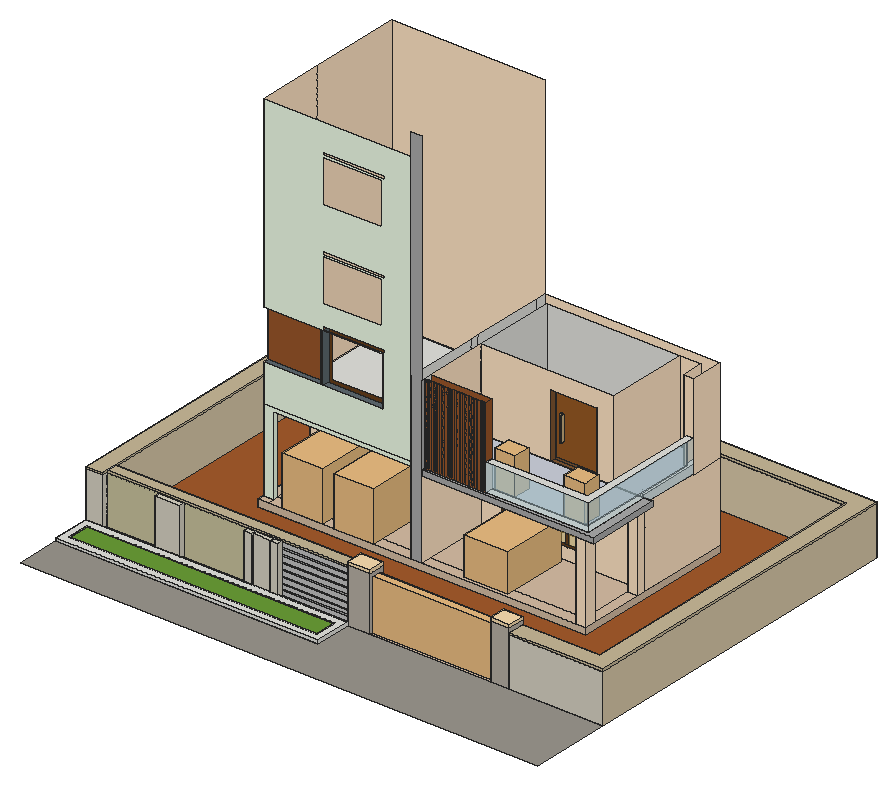
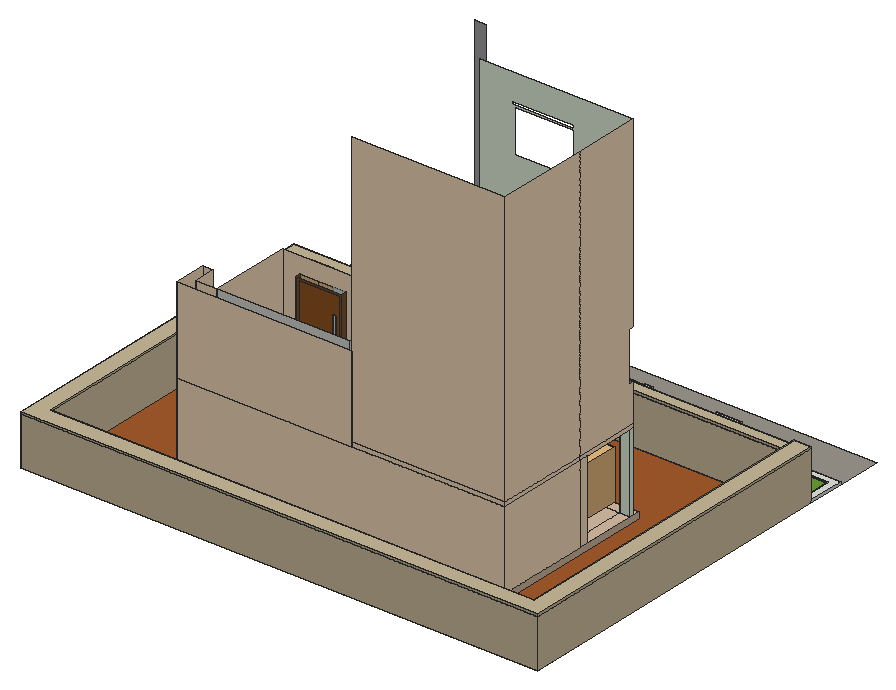
# SketchUp Ruby script. Lengths in inches.
U = 1.inch
M = Sketchup.active_model
def pt(a) = Geom::Point3d.new(a.map { |v| v * U })
def face(e, loops, mat)
  f = e.add_face(loops[0].map { |a| pt(a) })
  loops[1..].each { |l| e.add_face(l.map { |a| pt(a) }).erase! }
  f.material = f.back_material = mat if mat
  f
end
# faces: each face lists its corners as indices into pts; further lists are holes
def faces(e, pts, list, mat = nil) = list.each { |f| face(e, (f[0].is_a?(Array) ? f : [f]).map { |l| l.map { |i| pts[i] } }, mat) }
# xy, xz, yz: faces in a plane at the given z, y or x. An outline is a flat list of corners, or four numbers for a rectangle; further outlines are holes
def ring(l) = l.size == 4 ? [[l[0], l[1]], [l[2], l[1]], [l[2], l[3]], [l[0], l[3]]] : l.each_slice(2).to_a
def flat(e, list, mat, &to3) = list.each { |f| face(e, (f[0].is_a?(Array) ? f : [f]).map { |l| ring(l).map { |u, v| to3.(u, v) } }, mat) }
def xy(e, z, list, mat = nil) = flat(e, list, mat) { |x, y| [x, y, z] }
def xz(e, y, list, mat = nil) = flat(e, list, mat) { |x, z| [x, y, z] }
def yz(e, x, list, mat = nil) = flat(e, list, mat) { |y, z| [x, y, z] }
def lines(e, pts, list) = list.each { |a, b| e.add_line(pt(pts[a]), pt(pts[b])) }
# prism: a flat outline (further loops are holes) pulled along v
def prism(e, loops, v, mat = nil)
  f = face(e, loops, mat); d = Geom::Vector3d.new(v.map { |x| x * U })
  f.pushpull(f.normal.samedirection?(d) ? d.length : -d.length)
end
def box(e, o, s, mat = nil) = prism(e, [[o, [o[0] + s[0], o[1], o[2]], [o[0] + s[0], o[1] + s[1], o[2]], [o[0], o[1] + s[1], o[2]]]], [0, 0, s[2]], mat)
def at(x, y, z, deg = 0) = Geom::Transformation.translation(pt([x, y, z])) * Geom::Transformation.rotation(ORIGIN, Z_AXIS, deg.degrees)
def axes(o, x, y, z) = Geom::Transformation.new([*x, 0, *y, 0, *z, 0, *pt(o).to_a, 1])
def part(name) = M.definitions.add(name)
# library, detail: a bought-in or finely detailed component or shape, given as its bounding box
def library(name, o, s) = part(name).tap { |d| box(d.entities, o, s) }
def detail(e, o, s) = box(e.add_group.entities, o, s)
def put(e, d, t, mat = nil) = e.add_instance(d, t).tap { |i| i.material = mat if mat }
def group(e, t, mat = nil) = e.add_group.tap { |g| g.transformation = t; g.material = mat if mat }.entities
root = M.entities
M.materials.add("[0012_Bisque]").color = [255, 228, 196]
M.materials.add("[Carrera Marble]").color = [193, 193, 193]
M.materials.add("[Color M03]").color = [170, 170, 170]
M.materials.add("[Field Square Tile]").color = [217, 201, 169]
M.materials.add("[Formica Beige]").color = [249, 221, 176]
M.materials.add("[Formica Graystone]").color = [214, 209, 194]
M.materials.add("[Formica Laminate Light]").color = [213, 189, 164]
M.materials.add("[Formica Speckled Grey]1").color = [94, 105, 111]
M.materials.add("[Grass Dark Green]").color = [106, 157, 55]
M.materials.add("[Marble Carrara Floor Tile]").color = [204, 208, 219]
M.materials.add("[Quartz Light Brown]").color = [199, 184, 152]
M.materials.add("[Quartz Light Grey]").color = [251, 251, 252]
M.materials.add("[Rough Square Concrete Block]").color = [155, 151, 142]
M.materials.add("[Stone Coursed Rough]").color = [201, 195, 158]
M.materials.add("[Stone Masonry Multi]").color = [182, 175, 164]
M.materials.add("[Tile Limestone Large]1").color = [238, 251, 230]
M.materials.add("[Translucent Glass Gray]").color = [221, 178, 79]
M.materials["[Translucent Glass Gray]"].alpha = 0.5
M.materials.add("[Translucent Glass Safety]").color = [204, 235, 244]
M.materials["[Translucent Glass Safety]"].alpha = 0.42
M.materials.add("[Wood Bamboo]").color = [150, 89, 36]
M.materials.add("[Wood Cherry Original]").color = [152, 86, 42]
M.materials.add("[Wood Floor Light]").color = [204, 176, 127]
M.materials.add("[Wood Floor Parquet]").color = [102, 62, 27]
M.materials.add("[Wood Floor]").color = [127, 86, 50]
M.materials.add("[Wood Square Tile 01]").color = [164, 91, 44]
M.materials.add("[Wood Veneer 01]").color = [89, 52, 27]
M.materials.add("[Wood Veneer 02]").color = [119, 80, 57]
M.materials.add("[Wood Veneer 02]1").color = [190, 128, 91]
c1 = library("Gate_Lasercut_10ftx6ft_Kalil",[-0.15,-3.25,-0.15],[120,5.625,60.3])
c2 = library("skpE847",[-111.76,-15.01,0.76],[2.12,4.6,1.82])
c3 = part("car+1")
p = [[0,0,0],[1,0,0],[1,1,0]]
lines(c3.entities,p,[[0,1],[1,2],[2,0]])
put(c3.entities,c2,axes([-477.97,5140.8,-31.25],[0,46,0],[-46,0,0],[0,0,40.94]))
c4 = library("2015 Porsche Macan",[0.14,0.6,0.32],[90.05,184.43,65.58])
c5 = library("chau cay",[-24.34,-109.24,0],[56.46,62.58,79.69])
xy(root,0,[[[0,283.68,1655,516.81],[43.91,327.6,1611.08,472.9]],[0,516.81,0,2678.22,3268.59,2678.22,3268.59,516.81,2676.2,516.81,2676.2,622.2,3163.2,622.2,3163.2,2572.82,105.39,2572.82,105.39,516.81],[437.72,516.81,594.8,552.32],[997.32,516.81,1049.71,552.32],[1165.48,516.81,1213.51,552.32],
  [1655,516.81,1796.11,622.2],[2557.88,516.81,2676.2,622.2],[1049.71,525.25,1165.48,552.32],[105.39,552.32,1655,622.2],[560.3125,1175.74,2634.5,2234.7]])
xy(root,0,[[1796.11,516.81,2557.88,622.2]],"[Formica Laminate Light]")
xy(root,0,[[105.39,516.81,437.72,552.32],[594.8,516.81,997.32,552.32],[1049.71,516.81,1165.48,525.25],[1213.51,516.81,1655,552.32]],"[Quartz Light Grey]")
xy(root,0,[[0,0,0,283.68,1655,283.68,1655,516.81,3268.59,516.81,3268.59,0]],"[Rough Square Concrete Block]")
xy(root,0,[[[105.39,622.2,3163.2,2572.82],[560.3125,1175.74,2634.5,2234.7]]],"[Wood Square Tile 01]")
xy(root,12.4375,[[43.91,327.6,1611.08,472.9]],"[Grass Dark Green]")
xy(root,19,[[[0,283.68,1655,516.81],[43.91,327.6,1611.08,472.9]]])
xy(root,42.38,[[1529,1175.74,1597.41,1644.77],[2570.48,1175.74,2634.5,1247.68],[560.3125,1221.52,624.34,1247.68],[1504.0625,1221.52,1529,1247.68],[1504.0625,1247.68,1529,1644.77],
  [560.3125,1583.4,624.34,1644.77],[2570.48,1583.4,2634.5,1644.77],[560.3125,1644.77,560.3125,2234.7,2634.5,2234.7,2634.5,1644.77,2570.48,1644.77,2570.48,2162.77,624.34,2162.77,624.34,1644.77],[624.34,1644.77,624.34,1705.22,2570.48,1705.22,2570.48,1644.77,1498.82,1644.77,1498.82,1683.34,1254.8,1683.34,1254.8,1644.77],[624.34,1705.22,2570.48,2162.77]])
xy(root,42.38,[[560.3125,1175.74,624.34,1221.52],[624.34,1175.74,1529,1175.74,1529,1221.52,1504.0625,1221.52,1504.0625,1247.68,624.34,1247.68],[1597.41,1175.74,2570.48,1247.68],[560.3125,1247.68,624.34,1583.4],[624.34,1247.68,1504.0625,1247.68,1504.0625,1644.77,1498.82,1644.77,1498.82,1683.34,1254.8,1683.34,1254.8,1644.77,624.34,1644.77],
  [1597.41,1247.68,2570.48,1644.77],[2570.48,1247.68,2634.5,1583.4]],"[Formica Laminate Light]")
xy(root,305.6875,[[0,516.81,0,2678.22,3268.59,2678.22,3268.59,516.81,2676.2,516.81,2676.2,622.2,3163.2,622.2,3163.2,2572.82,105.39,2572.82,105.39,516.81],[105.39,552.32,1655,622.2]])
xy(root,305.6875,[[437.72,516.81,594.8,552.32],[997.32,516.81,1049.71,552.32],[1165.48,516.81,1213.51,552.32],[1049.71,525.25,1165.48,552.32]],"[Formica Graystone]")
xy(root,318.25,[[0,516.81,105.39,516.81,105.39,2572.82,3163.2,2572.82,3163.2,622.2,2676.2,622.2,2676.2,516.81,3268.59,516.81,3268.59,2678.22,0,2678.22],[105.39,552.32,1655,622.2]],"[Quartz Light Brown]")
xy(root,342.3125,[[1655,516.81,1796.11,622.2],[2557.88,516.81,2676.2,622.2]])
xy(root,362.6875,[[1655,516.81,1796.11,622.2],[2557.88,516.81,2676.2,622.2]],"[Formica Beige]")
xy(root,463.2,[[1254.8,1644.77,1498.82,1683.34]],"[0012_Bisque]")
xy(root,535.87,[[2570.48,1175.74,2634.5,1247.68],[2634.5,1175.74,2683.95,1247.68],[560.3125,1583.4,560.3125,2234.7,1529,2234.7,1529,1644.77,624.34,1644.77,624.34,1583.4],[2570.48,1583.4,2634.5,1644.77],[2634.5,1583.4,2683.95,1644.77],
  [1597.41,1644.77,2570.48,2162.77]])
xy(root,535.87,[[1597.41,1175.74,1597.41,1644.77,2570.48,1644.77,2570.48,1583.4,2683.95,1583.4,2683.95,1247.68,2570.48,1247.68,2570.48,1175.74],[624.34,1221.52,1504.0625,1644.77]],"[0012_Bisque]")
xy(root,535.87,[[560.3125,1247.68,624.34,1583.4]],"[Tile Limestone Large]1")
xy(root,561.43,[[560.3125,1221.52,1529,2234.7]])
xy(root,569.39,[[1597.41,1197.49,1985.07,1247.68],[1985.07,1197.49,1985.07,1247.68,2590.83,1247.68,2590.83,1644.77,2634.5,1644.77,2634.5,1197.49],[1597.41,1644.77,1597.41,2162.77,2438.87,2162.77,2438.87,1644.77,2328.14,1644.77,2328.14,1674.71,2038.61,1674.71,2038.61,1644.77]])
xy(root,569.39,[[1597.41,1175.74,2683.95,1175.74,2683.95,1644.77,2634.5,1644.77,2634.5,1197.49,1597.41,1197.49]],"[Color M03]")
xy(root,569.39,[[1597.41,1247.68,2590.83,1644.77],[2438.87,1644.77,2590.83,1644.77,2590.83,2027.6,2570.48,2027.6,2570.48,2162.77,2438.87,2162.77]],"[Marble Carrara Floor Tile]")
xy(root,569.39,[[2038.61,1644.77,2328.14,1674.71]],"[Wood Floor]")
xy(root,740.5625,[[1985.07,1197.49,2634.5,1197.49,2634.5,2027.6,2590.83,2027.6,2590.83,1247.68,1985.07,1247.68]])
xy(root,798.61,[[560.3125,1221.52,922.73,1257.65],[937.5625,1221.52,1314.8125,1263.33]],"[Formica Speckled Grey]1")
xz(root,283.68,[[0,0,1655,19]])
xz(root,327.6,[[43.91,12.4375,1611.08,19]])
xz(root,327.6,[[43.91,0,1611.08,12.4375]],"[Grass Dark Green]")
xz(root,472.9,[[43.91,12.4375,1611.08,19]])
xz(root,472.9,[[43.91,0,1611.08,12.4375]],"[Grass Dark Green]")
xz(root,516.81,[[0,0,105.39,19],[105.39,0,437.72,19],[437.72,0,594.8,19],[594.8,0,997.32,19],[997.32,0,1049.71,19],
  [1049.71,0,1165.48,19],[1165.48,0,1213.51,19],[1213.51,0,1655,19]])
xz(root,516.81,[[1655,342.3125,1796.11,362.6875],[2557.88,342.3125,2676.2,362.6875]],"[Formica Beige]")
xz(root,516.81,[[2676.2,0,3268.59,305.6875],[0,19,105.39,305.6875],[437.72,19,594.8,305.6875],[997.32,19,1049.71,305.6875],[1165.48,19,1213.51,305.6875]],"[Formica Graystone]")
xz(root,516.81,[[0,305.6875,105.39,318.25],[2676.2,305.6875,3268.59,318.25]],"[Quartz Light Brown]")
xz(root,516.81,[[1655,0,1796.11,342.3125],[2557.88,0,2676.2,342.3125]],"[Stone Masonry Multi]")
xz(root,525.25,[[1049.71,0,1165.48,305.6875]],"[Formica Graystone]")
xz(root,552.32,[[437.72,0,594.8,305.6875],[997.32,0,1049.71,305.6875],[1049.71,0,1165.48,305.6875],[1165.48,0,1213.51,305.6875]])
xz(root,552.32,[[1213.51,0,1655,29.67],[1213.51,36.26,1655,62.625],[1213.51,69.17,1655,102.125],[1213.51,108.61,1655,141.5625],[1213.51,151.05,1655,184],
  [1213.51,191.55,1655,224.5],[1213.51,232.55,1655,265.5],[1213.51,272.74,1655,305.6875]],"[Carrera Marble]")
xz(root,552.32,[[1213.51,29.67,1655,36.26],[1213.51,62.625,1655,69.17],[1213.51,102.125,1655,108.61],[1213.51,141.5625,1655,151.05],[1213.51,184,1655,191.55],
  [1213.51,224.5,1655,232.55],[1213.51,265.5,1655,272.74]],"[Color M03]")
xz(root,552.32,[[105.39,305.6875,1655,318.25]],"[Quartz Light Brown]")
xz(root,552.32,[[105.39,0,437.72,305.6875],[594.8,0,997.32,305.6875]],"[Stone Coursed Rough]")
xz(root,622.2,[[105.39,0,1655,305.6875],[2676.2,0,3163.2,305.6875]],"[Field Square Tile]")
xz(root,622.2,[[1655,342.3125,1796.11,362.6875],[2557.88,342.3125,2676.2,362.6875]],"[Formica Beige]")
xz(root,622.2,[[105.39,305.6875,1655,318.25],[2676.2,305.6875,3163.2,318.25]],"[Quartz Light Brown]")
xz(root,622.2,[[1655,0,1796.11,342.3125],[2557.88,0,2676.2,342.3125]],"[Stone Masonry Multi]")
xz(root,1175.74,[[2570.48,42.38,2634.5,535.87]],"[0012_Bisque]")
xz(root,1175.74,[[1529,42.38,1597.41,2461.1],[1597.41,535.87,2683.95,569.39]],"[Color M03]")
xz(root,1175.74,[[560.3125,0,2634.5,42.38]],"[Formica Laminate Light]")
xz(root,1197.49,[[1985.07,569.39,2634.5,740.5625]],"[Translucent Glass Safety]")
xz(root,1197.49,[[1597.41,569.39,1608.66,1077.79],[1608.66,569.39,1611.91,1077.79],[1611.91,569.39,1623.16,1077.79],[1623.16,569.39,1626.47,1077.79],[1626.47,569.39,1637.72,1077.79],
  [1637.72,569.39,1641.03,1077.79],[1641.03,569.39,1652.28,1077.79],[1652.28,569.39,1655.59,1077.79],[1655.59,569.39,1666.85,1077.79],[1666.85,569.39,1670.16,1077.79],
  [1670.16,569.39,1681.41,1077.79],[1681.41,569.39,1684.72,1077.79],[1684.72,569.39,1695.97,1077.79],[1695.97,569.39,1699.28,1077.79],[1699.28,569.39,1710.53,1077.79],
  [1710.53,569.39,1713.84,1077.79],[1713.84,569.39,1725.1,1077.79],[1725.1,569.39,1728.41,1077.79],[1728.41,569.39,1739.66,1077.79],[1739.66,569.39,1742.97,1077.79],
  [1742.97,569.39,1754.22,1077.79],[1754.22,569.39,1757.53,1077.79],[1757.53,569.39,1768.78,1077.79],[1768.78,569.39,1772.09,1077.79],[1772.09,569.39,1783.35,1077.79],
  [1783.35,569.39,1786.66,1077.79],[1786.66,569.39,1797.91,1077.79],[1797.91,569.39,1801.22,1077.79],[1801.22,569.39,1812.47,1077.79],[1812.47,569.39,1815.78,1077.79],
  [1815.78,569.39,1827.03,1077.79],[1827.03,569.39,1830.34,1077.79],[1830.34,569.39,1841.6,1077.79],[1841.6,569.39,1844.91,1077.79],[1844.91,569.39,1856.16,1077.79],
  [1856.16,569.39,1859.47,1077.79],[1859.47,569.39,1870.72,1077.79],[1870.72,569.39,1874.03,1077.79],[1874.03,569.39,1885.28,1077.79],[1885.28,569.39,1889.22,1077.79],
  [1889.22,569.39,1900.47,1077.79],[1900.47,569.39,1904.41,1077.79],[1904.41,569.39,1915.66,1077.79],[1915.66,569.39,1919.59,1077.79],[1919.59,569.39,1930.85,1077.79],
  [1930.85,569.39,1934.78,1077.79],[1934.78,569.39,1946.03,1077.79],[1946.03,569.39,1949.97,1077.79],[1949.97,569.39,1961.22,1077.79],[1961.22,569.39,1963.53,1077.79],
  [1963.53,569.39,1971.7,1077.79],[1971.7,569.39,1974.78,1077.79],[1974.78,569.39,1985.07,1077.79]],"[Wood Cherry Original]")
xz(root,1221.52,[[560.3125,42.38,624.34,42.38,624.34,535.87,1504.0625,535.87,1504.0625,42.38,1529,42.38,1529,561.43,560.3125,561.43],[[560.3125,561.43,1529,561.43,1529,2288.72,560.3125,2288.72,560.3125,1108.67,1314.8125,1108.67,1314.8125,798.61,560.3125,798.61],[937.5625,1262.3,1307.26,1530.73],[937.5625,1822.8,1307.26,2091.23],[934.42,1113.51,1328.79,1133.63],[934.42,1536.95,1328.79,1557.07],[934.42,2101.01,1328.79,2121.13]]],"[Tile Limestone Large]1")
xz(root,1221.52,[[922.73,798.61,937.5625,1108.67]],"[Wood Veneer 02]1")
xz(root,1247.68,[[2570.48,42.38,2634.5,535.87]],"[0012_Bisque]")
xz(root,1247.68,[[560.3125,42.38,624.34,535.87]],"[Tile Limestone Large]1")
xz(root,1247.68,[[1985.07,569.39,2590.83,740.5625]],"[Translucent Glass Safety]")
xz(root,1247.68,[[1597.41,569.39,1985.07,1077.79]],"[Wood Cherry Original]")
xz(root,1257.65,[[560.3125,798.61,922.73,1108.67]],"[Wood Cherry Original]")
xz(root,1263.33,[[[937.5625,798.61,1314.8125,1108.67],[959.46,820.51,1292.91,1086.78]]],"[Wood Floor Parquet]")
xz(root,1583.4,[[560.3125,42.38,624.34,535.87],[2570.48,42.38,2634.5,535.87]],"[0012_Bisque]")
xz(root,1644.77,[[1504.0625,42.38,1529,535.87],[2570.48,42.38,2634.5,535.87],[1597.41,535.87,2570.48,569.39],[2570.48,535.87,2634.5,569.39],[2634.5,535.87,2683.95,569.39]])
xz(root,1644.77,[[[624.34,42.38,1254.8,42.38,1254.8,463.2,1498.82,463.2,1498.82,42.38,1504.0625,42.38,1504.0625,535.87,624.34,535.87],[913.02,202.39,1188.92,456.59]],[[1597.41,42.38,2570.48,535.87],[1722.09,114.49,2308.54,441.42]],[1597.41,569.39,2038.61,569.39,2038.61,972.31,2328.14,972.31,2328.14,569.39,2438.87,569.39,2438.87,1077.79,1597.41,1077.79]],"[0012_Bisque]")
xz(root,1644.77,[[1741.6,132.47,1864.16,423.4375],[1882.99,132.47,1999.39,423.4375],[2018.21,132.47,2134.79,423.4375],[2153.62,132.47,2289.03,423.4375],[929.18,217.28,1037.92,441.7],
  [1062.5,217.28,1172.76,441.7]],"[Translucent Glass Gray]")
xz(root,1644.77,[[[1722.09,114.49,2308.54,441.42],[1741.6,132.47,2289.03,423.4375]],[1864.16,132.47,1882.99,423.4375],[1999.39,132.47,2018.21,423.4375],[2134.79,132.47,2153.62,423.4375]],"[Wood Floor Parquet]")
xz(root,1644.77,[[[913.02,202.39,1188.92,456.59],[929.18,217.28,1172.76,441.7]],[1037.92,217.28,1062.5,441.7]],"[Wood Veneer 02]")
xz(root,1663.21,[[2085.88,679.48,2087.99,679.76,2089.96,680.57,2091.65,681.87,2092.95,683.56,2093.76,685.52,2094.04,687.63,2094.04,836.07,2093.76,838.18,2092.95,840.15,2091.65,841.84,2089.96,843.14,2087.99,843.95,2085.88,844.23,2083.77,843.95,2081.8,843.14,2080.12,841.84,2078.82,840.15,2078,838.18,2077.73,836.07,2077.73,687.63,2078,685.52,2078.82,683.56,2080.12,681.87,2081.8,680.57,2083.77,679.76]],"[Wood Floor Light]")
xz(root,1674.71,[[2085.88,679.48,2083.77,679.76,2081.8,680.57,2080.12,681.87,2078.82,683.56,2078,685.52,2077.73,687.63,2077.73,836.07,2078,838.18,2078.82,840.15,2080.12,841.84,2081.8,843.14,2083.77,843.95,2085.88,844.23,2087.99,843.95,2089.96,843.14,2091.65,841.84,2092.95,840.15,2093.76,838.18,2094.04,836.07,2094.04,687.63,2093.76,685.52,2092.95,683.56,2091.65,681.87,2089.96,680.57,2087.99,679.76]])
xz(root,1674.71,[[[2054.85,584.34,2311.91,957.36],[2085.88,679.48,2083.77,679.76,2081.8,680.57,2080.12,681.87,2078.82,683.56,2078,685.52,2077.73,687.63,2077.73,836.07,2078,838.18,2078.82,840.15,2080.12,841.84,2081.8,843.14,2083.77,843.95,2085.88,844.23,2087.99,843.95,2089.96,843.14,2091.65,841.84,2092.95,840.15,2093.76,838.18,2094.04,836.07,2094.04,687.63,2093.76,685.52,2092.95,683.56,2091.65,681.87,2089.96,680.57,2087.99,679.76]]],"[Wood Bamboo]")
xz(root,1674.71,[[[2038.61,569.39,2328.14,972.31],[2054.85,584.34,2311.91,957.36]]],"[Wood Floor]")
xz(root,1683.34,[[[1254.8,42.38,1498.82,463.2],[1272.26,58.47,1481.36,447.11]],[1272.26,58.47,1481.36,447.11]],"[Wood Veneer 01]")
xz(root,2027.6,[[2570.48,569.39,2590.83,569.39,2590.83,740.5625,2634.5,740.5625,2634.5,1077.79,2570.48,1077.79]],"[0012_Bisque]")
xz(root,2162.77,[[1597.41,535.87,2570.48,569.39],[1597.41,569.39,2438.87,1077.79]])
xz(root,2162.77,[[2438.87,569.39,2570.48,1077.79]],"[0012_Bisque]")
xz(root,2234.7,[[560.3125,42.38,2634.5,535.87],[560.3125,535.87,1529,561.43],[1529,535.87,2634.5,1077.79],[560.3125,561.43,1529,2288.72]],"[0012_Bisque]")
xz(root,2234.7,[[560.3125,0,2634.5,42.38]],"[Formica Laminate Light]")
xz(root,2572.82,[[105.39,0,3163.2,305.6875]],"[Field Square Tile]")
xz(root,2572.82,[[105.39,305.6875,3163.2,318.25]],"[Quartz Light Brown]")
xz(root,2678.22,[[0,0,3268.59,305.6875]],"[Field Square Tile]")
xz(root,2678.22,[[0,305.6875,3268.59,318.25]],"[Quartz Light Brown]")
yz(root,0,[[283.68,0,516.81,19]])
yz(root,0,[[516.81,0,2678.22,305.6875]],"[Field Square Tile]")
yz(root,0,[[516.81,305.6875,2678.22,318.25]],"[Quartz Light Brown]")
yz(root,43.91,[[327.6,12.4375,472.9,19]])
yz(root,43.91,[[327.6,0,472.9,12.4375]],"[Grass Dark Green]")
yz(root,105.39,[[552.32,0,622.2,305.6875],[552.32,305.6875,622.2,318.25]])
yz(root,105.39,[[622.2,0,2572.82,305.6875]],"[Field Square Tile]")
yz(root,105.39,[[516.81,0,552.32,305.6875]],"[Formica Graystone]")
yz(root,105.39,[[516.81,305.6875,552.32,318.25],[622.2,305.6875,2572.82,318.25]],"[Quartz Light Brown]")
yz(root,437.72,[[516.81,0,552.32,305.6875]],"[Formica Graystone]")
yz(root,560.3125,[[1583.4,42.38,1644.77,535.87],[1644.77,42.38,2234.7,535.87],[1221.52,535.87,1644.77,561.43],[1644.77,535.87,2234.7,561.43],[1221.52,561.43,1221.52,798.61,1257.65,798.61,1257.65,1108.67,1221.52,1108.67,1221.52,2288.72,1644.77,2288.72,1644.77,561.43],
  [1644.77,561.43,2234.7,2288.72]],"[0012_Bisque]")
yz(root,560.3125,[[1175.74,0,2234.7,42.38]],"[Formica Laminate Light]")
yz(root,560.3125,[[1221.52,42.38,1247.68,535.87]],"[Tile Limestone Large]1")
yz(root,594.8,[[516.81,0,552.32,305.6875]],"[Formica Graystone]")
yz(root,624.34,[[1583.4,42.38,1644.77,535.87]],"[0012_Bisque]")
yz(root,624.34,[[1221.52,42.38,1247.68,535.87]],"[Tile Limestone Large]1")
yz(root,922.73,[[1221.52,798.61,1257.65,1108.67]],"[Wood Veneer 02]1")
yz(root,937.5625,[[1221.52,798.61,1263.33,1108.67]],"[Formica Speckled Grey]1")
yz(root,997.32,[[516.81,0,552.32,305.6875]],"[Formica Graystone]")
yz(root,1049.71,[[525.25,0,552.32,305.6875]])
yz(root,1049.71,[[516.81,0,525.25,305.6875]],"[Formica Graystone]")
yz(root,1165.48,[[525.25,0,552.32,305.6875]])
yz(root,1165.48,[[516.81,0,525.25,305.6875]],"[Formica Graystone]")
yz(root,1213.51,[[516.81,0,552.32,305.6875]],"[Formica Graystone]")
yz(root,1254.8,[[1644.77,42.38,1683.34,463.2]],"[0012_Bisque]")
yz(root,1314.8125,[[1221.52,798.61,1263.33,1108.67]],"[Formica Speckled Grey]1")
yz(root,1498.82,[[1644.77,42.38,1683.34,463.2]],"[0012_Bisque]")
yz(root,1504.0625,[[1221.52,42.38,1644.77,535.87]],"[0012_Bisque]")
yz(root,1529,[[1221.52,42.38,1644.77,535.87],[1221.52,535.87,1705.22,561.43],[1705.22,535.87,2162.77,561.43],[2162.77,535.87,2234.7,561.43],[1221.52,561.43,1644.77,1077.79],
  [1644.77,561.43,1705.22,1077.79],[1705.22,561.43,2162.77,1077.79],[2162.77,561.43,2234.7,1077.79]])
yz(root,1529,[[1175.74,42.38,1221.52,535.87],[1175.74,535.87,1221.52,561.43],[1175.74,561.43,1221.52,1077.79]],"[Color M03]")
yz(root,1597.41,[[1175.74,535.87,1247.68,569.39],[1247.68,535.87,1644.77,569.39],[1644.77,535.87,2162.77,569.39],[1197.49,569.39,1247.68,1077.79],[1644.77,569.39,2162.77,1077.79]])
yz(root,1597.41,[[1175.74,42.38,1644.77,535.87],[1247.68,569.39,1644.77,1077.79]],"[0012_Bisque]")
yz(root,1597.41,[[1175.74,569.39,1197.49,1077.79]],"[Color M03]")
yz(root,1611.08,[[327.6,12.4375,472.9,19]])
yz(root,1611.08,[[327.6,0,472.9,12.4375]],"[Grass Dark Green]")
yz(root,1655,[[283.68,0,516.81,19],[552.32,0,622.2,305.6875],[552.32,305.6875,622.2,318.25]])
yz(root,1655,[[516.81,342.3125,622.2,362.6875]],"[Formica Beige]")
yz(root,1655,[[516.81,0,516.81,342.3125,622.2,342.3125,622.2,318.25,552.32,318.25,552.32,0]],"[Stone Masonry Multi]")
yz(root,1796.11,[[516.81,342.3125,622.2,362.6875]],"[Formica Beige]")
yz(root,1796.11,[[516.81,0,622.2,342.3125]],"[Stone Masonry Multi]")
yz(root,1985.07,[[1197.49,569.39,1247.68,740.5625]])
yz(root,1985.07,[[1197.49,740.5625,1247.68,1077.79]],"[Wood Cherry Original]")
yz(root,2038.61,[[1644.77,569.39,1674.71,972.31]],"[Wood Floor]")
yz(root,2077.73,[[1663.21,687.63,1674.71,836.07]],"[Wood Floor Light]")
yz(root,2094.04,[[1663.21,687.63,1674.71,836.07]],"[Wood Floor Light]")
yz(root,2328.14,[[1644.77,569.39,1674.71,972.31]],"[Wood Floor]")
yz(root,2438.87,[[1644.77,569.39,2162.77,1077.79]],"[0012_Bisque]")
yz(root,2557.88,[[516.81,342.3125,622.2,362.6875]],"[Formica Beige]")
yz(root,2557.88,[[516.81,0,622.2,342.3125]],"[Stone Masonry Multi]")
yz(root,2570.48,[[1644.77,42.38,1705.22,535.87],[1705.22,42.38,2162.77,535.87]])
yz(root,2570.48,[[1175.74,42.38,1247.68,535.87],[1583.4,42.38,1644.77,535.87],[2027.6,569.39,2162.77,1077.79]],"[0012_Bisque]")
yz(root,2590.83,[[1247.68,569.39,2027.6,740.5625]],"[Translucent Glass Safety]")
yz(root,2634.5,[[1175.74,42.38,1247.68,535.87],[1583.4,42.38,1644.77,535.87],[1644.77,42.38,2234.7,535.87],[2027.6,535.87,2234.7,1077.79]],"[0012_Bisque]")
yz(root,2634.5,[[1175.74,0,2234.7,42.38]],"[Formica Laminate Light]")
yz(root,2634.5,[[1644.77,535.87,2027.6,535.87,2027.6,740.5625,1197.49,740.5625,1197.49,569.39,1644.77,569.39]],"[Translucent Glass Safety]")
yz(root,2676.2,[[516.81,0,622.2,305.6875],[516.81,305.6875,622.2,318.25]])
yz(root,2676.2,[[516.81,342.3125,622.2,362.6875]],"[Formica Beige]")
yz(root,2676.2,[[516.81,318.25,622.2,342.3125]],"[Stone Masonry Multi]")
yz(root,2683.95,[[1175.74,535.87,1644.77,569.39]],"[Color M03]")
yz(root,3163.2,[[622.2,0,2572.82,305.6875]],"[Field Square Tile]")
yz(root,3163.2,[[622.2,305.6875,2572.82,318.25]],"[Quartz Light Brown]")
yz(root,3268.59,[[516.81,0,2678.22,305.6875]],"[Field Square Tile]")
yz(root,3268.59,[[516.81,305.6875,2678.22,318.25]],"[Quartz Light Brown]")
p = [[2083.77,1674.71,679.76],[2085.88,1674.71,679.48],[2085.88,1663.21,679.48],[2083.77,1663.21,679.76],[2087.99,1674.71,679.76],[2087.99,1663.21,679.76],
  [2081.8,1674.71,680.57],[2081.8,1663.21,680.57],[2089.96,1674.71,680.57],[2089.96,1663.21,680.57],[2080.12,1674.71,681.87],[2080.12,1663.21,681.87],
  [2091.65,1674.71,681.87],[2091.65,1663.21,681.87],[2078.82,1674.71,683.56],[2078.82,1663.21,683.56],[2092.95,1674.71,683.56],[2092.95,1663.21,683.56],
  [2078,1674.71,685.52],[2078,1663.21,685.52],[2093.76,1674.71,685.52],[2093.76,1663.21,685.52],[2077.73,1674.71,687.63],[2077.73,1663.21,687.63],
  [2094.04,1674.71,687.63],[2094.04,1663.21,687.63],[624.34,2162.77,42.38],[624.34,2162.77,535.87],[624.34,1705.22,42.38],[624.34,1705.22,535.87],
  [2570.48,1705.22,535.87],[2570.48,1705.22,569.39]]
faces(root,p,[[0,1,2,3],[1,4,5,2],[6,0,3,7],[4,8,9,5],[10,6,7,11],[8,12,13,9],[14,10,11,15],[12,16,17,13],
  [18,14,15,19],[16,20,21,17],[22,18,19,23],[20,24,25,21]],"[Wood Floor Light]")
lines(root,p,[[26,27],[28,29],[30,31]])
put(root,c1,axes([1796.11,564.26,0.4],[6.2607,0,0],[0,9.15712,0],[0,0,5.30156]))
put(root,c3,axes([1846.78,1616.43,42.38],[0,-1.9635,0],[2.85,0,0],[0,0,3.2]))
put(root,c4,axes([1038.14,1174.25,40.87],[2.8122,0,0],[0,2.46,0],[0,0,4.75013]))
put(root,c4,axes([713.8,1175.74,42.23],[2.8122,0,0],[0,2.46,0],[0,0,4.75013]))
put(root,c5,axes([2490.79,1445.37,569.39],[2.3,0,0],[0,1.769,0],[0,0,2.9044]))
put(root,c5,axes([2051.04,1445.37,569.39],[2.3,0,0],[0,1.769,0],[0,0,2.9044]))
